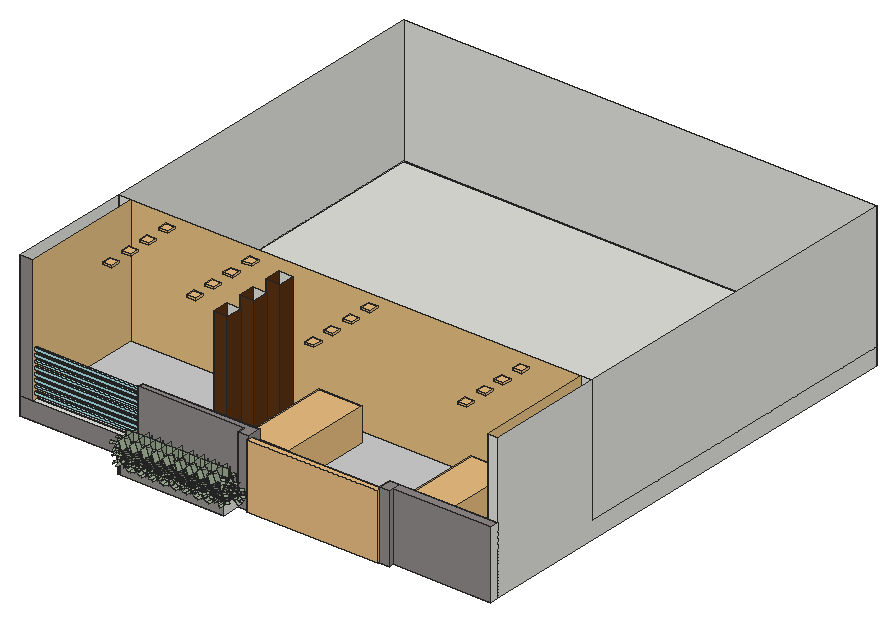
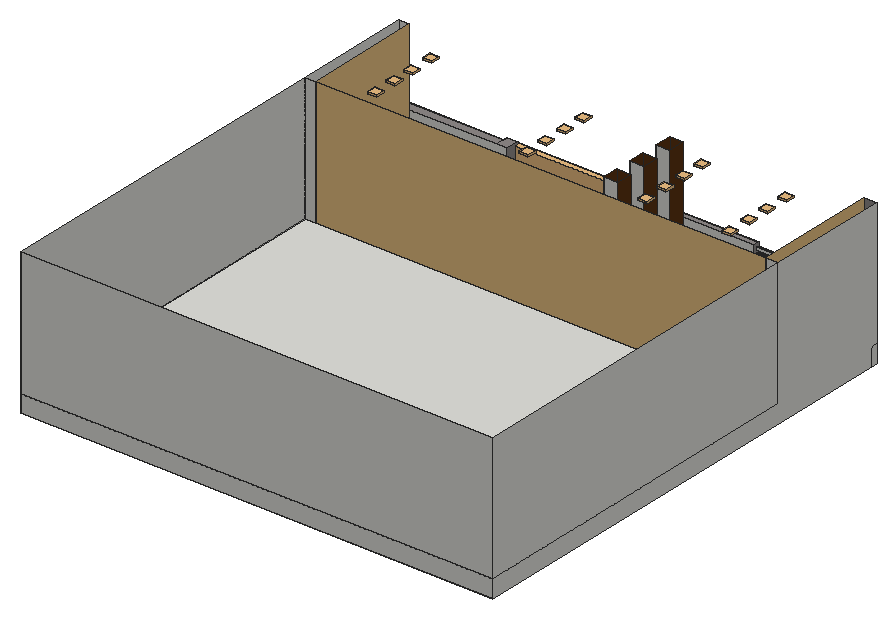
# SketchUp Ruby script. Lengths in inches.
U = 1.inch
M = Sketchup.active_model
def pt(a) = Geom::Point3d.new(a.map { |v| v * U })
def face(e, loops, mat)
  f = e.add_face(loops[0].map { |a| pt(a) })
  loops[1..].each { |l| e.add_face(l.map { |a| pt(a) }).erase! }
  f.material = f.back_material = mat if mat
  f
end
# faces: each face lists its corners as indices into pts; further lists are holes
def faces(e, pts, list, mat = nil) = list.each { |f| face(e, (f[0].is_a?(Array) ? f : [f]).map { |l| l.map { |i| pts[i] } }, mat) }
# xy, xz, yz: faces in a plane at the given z, y or x. An outline is a flat list of corners, or four numbers for a rectangle; further outlines are holes
def ring(l) = l.size == 4 ? [[l[0], l[1]], [l[2], l[1]], [l[2], l[3]], [l[0], l[3]]] : l.each_slice(2).to_a
def flat(e, list, mat, &to3) = list.each { |f| face(e, (f[0].is_a?(Array) ? f : [f]).map { |l| ring(l).map { |u, v| to3.(u, v) } }, mat) }
def xy(e, z, list, mat = nil) = flat(e, list, mat) { |x, y| [x, y, z] }
def xz(e, y, list, mat = nil) = flat(e, list, mat) { |x, z| [x, y, z] }
def yz(e, x, list, mat = nil) = flat(e, list, mat) { |y, z| [x, y, z] }
def lines(e, pts, list) = list.each { |a, b| e.add_line(pt(pts[a]), pt(pts[b])) }
# prism: a flat outline (further loops are holes) pulled along v
def prism(e, loops, v, mat = nil)
  f = face(e, loops, mat); d = Geom::Vector3d.new(v.map { |x| x * U })
  f.pushpull(f.normal.samedirection?(d) ? d.length : -d.length)
end
def box(e, o, s, mat = nil) = prism(e, [[o, [o[0] + s[0], o[1], o[2]], [o[0] + s[0], o[1] + s[1], o[2]], [o[0], o[1] + s[1], o[2]]]], [0, 0, s[2]], mat)
def at(x, y, z, deg = 0) = Geom::Transformation.translation(pt([x, y, z])) * Geom::Transformation.rotation(ORIGIN, Z_AXIS, deg.degrees)
def axes(o, x, y, z) = Geom::Transformation.new([*x, 0, *y, 0, *z, 0, *pt(o).to_a, 1])
def part(name) = M.definitions.add(name)
# library, detail: a bought-in or finely detailed component or shape, given as its bounding box
def library(name, o, s) = part(name).tap { |d| box(d.entities, o, s) }
def detail(e, o, s) = box(e.add_group.entities, o, s)
def put(e, d, t, mat = nil) = e.add_instance(d, t).tap { |i| i.material = mat if mat }
def group(e, t, mat = nil) = e.add_group.tap { |g| g.transformation = t; g.material = mat if mat }.entities
root = M.entities
M.materials.add("Generic").color = [90, 50, 18]
M.materials.add("Generic\#5").color = [233, 194, 132]
M.materials.add("Generic\#7").color = [171, 227, 232]
M.materials.add("[Carrera Marble]").color = [207, 207, 207]
M.materials.add("[Granite Light Gray]").color = [149, 148, 144]
M.materials.add("[Stone Marble]").color = [143, 138, 136]
M.materials.add("hymenocallis littoralis").color = [156, 172, 146]
c1 = part("Group\#856")
xy(c1.entities,7.38,[[0,0,5.5,15.91]],"hymenocallis littoralis")
p = [[5.5,28.78,0],[5.5,26.79,3.44],[0,26.79,3.44],[0,28.78,0],[0,23.75,6],[5.5,23.75,6],
  [0,15.91,7.38],[5.5,15.91,7.38]]
faces(c1.entities,p,[[0,1,2,3],[4,2,1,5],[6,4,5,7]],"hymenocallis littoralis")
c2 = part("Group\#854")
xy(c2.entities,7.38,[[0,0,5.5,15.91],[0,15.91,5.5,23.87]],"hymenocallis littoralis")
p = [[5.5,31.07,4.3],[5.5,27.74,6.47],[0,27.74,6.47],[0,31.07,4.3],[0,23.87,7.38],[5.5,23.87,7.38]]
faces(c2.entities,p,[[0,1,2,3],[4,2,1,5]],"hymenocallis littoralis")
c3 = part("Group\#857")
xy(c3.entities,7.38,[[0,0,5.6,15.91]],"hymenocallis littoralis")
p = [[5.6,28.78,0],[5.6,26.79,3.44],[0,26.79,3.44],[0,28.78,0],[0,23.75,6],[5.6,23.75,6],
  [0,15.91,7.38],[5.6,15.91,7.38]]
faces(c3.entities,p,[[0,1,2,3],[4,2,1,5],[6,4,5,7]],"hymenocallis littoralis")
c4 = part("Group\#855")
put(c4.entities,c2,axes([6.09,8.57,-0.52],[0.446,0.85617,0.26089],[-0.18444,-0.19731,0.96283],[0.87582,-0.47754,0.0699]))
put(c4.entities,c2,axes([6.29,7.28,-1.71],[0.37058,0.92707,-0.05667],[-0.32382,0.19004,0.99128],[0.87712,-0.32925,0.34964]))
put(c4.entities,c2,axes([11.04,16.14,-0.7],[1,0,0],[0,0.16628,1.02662],[0,-1.18456,0.19186]))
c5 = part("Group\#860")
put(c5.entities,c1,axes([24.57,32.05,-1.76],[0.9552,-0.22102,-0.19681],[0.4036,0.95545,0.88585],[-0.00568,-0.67859,0.7345]))
put(c5.entities,c1,axes([23.95,29.24,-2.4],[0,1,0],[-0.76041,0,0.64945],[0.64945,0,0.76041]))
put(c5.entities,c1,axes([24.22,24.72,-0.48],[-0.70711,0.70711,0],[-0.32757,-0.32757,0.80237],[0.61237,0.61237,0.5]))
put(c5.entities,c2,axes([20.66,37.22,-0.63],[1.12361,0.03262,0.39091],[-0.43499,0.29739,0.78777],[0.09852,-1.27434,0.37535]))
put(c5.entities,c1,axes([28.75,24.45,-2.4],[-1,0,0],[0,-0.76041,0.64945],[0,0.64945,0.76041]))
put(c5.entities,c3,axes([30.4,30.98,-3.7],[0.65676,-0.72002,0.22414],[0.55667,0.66341,0.5],[-0.50871,-0.20361,0.83652]))
put(c5.entities,c3,axes([32.41,29.61,-3.7],[0.04029,-0.97372,0.22414],[0.85287,0.15038,0.5],[-0.52057,0.17102,0.83652]))
put(c5.entities,c1,axes([31.89,25.85,-1.76],[-0.92056,0.33739,-0.19681],[-0.5186,-0.89824,0.88585],[0.08952,0.67268,0.7345]))
put(c5.entities,c1,axes([25.55,34.78,-0.48],[0.86603,0.5,0],[-0.25,0.43301,0.86603],[0.43301,-0.75,0.5]))
put(c5.entities,c3,axes([20.4,16.9375,-8.07],[-0.70711,0.70711,0],[-0.35754,-0.35754,0.65422],[1.3987,1.3987,1.52882]))
put(c5.entities,c1,axes([32.86,34.14,-0.48],[0.76604,-0.64279,0],[0.32139,0.38302,0.86603],[-0.55667,-0.66341,0.5]))
put(c5.entities,c1,axes([27.15,34.7,-0.1],[0.82472,-0.17528,-0.53769],[0.53769,0.53769,0.64945],[0.17528,-0.82472,0.53769]))
put(c5.entities,c1,axes([33.58,28.77,-2.4],[0,-1,0],[0.76041,0,0.64945],[-0.64945,0,0.76041]))
put(c5.entities,c1,axes([26.43,23.87,-2.81],[-0.75126,0.04415,0.65853],[0.53769,-0.53769,0.64945],[0.38276,0.84199,0.3802]))
put(c5.entities,c1,axes([28.78,23.98,-2.4],[-1,0,0],[0,-0.76041,0.64945],[0,0.64945,0.76041]))
put(c5.entities,c1,axes([25.39,25.38,-2.4],[-0.70711,0.70711,0],[-0.53769,-0.53769,0.64945],[0.45923,0.45923,0.76041]))
put(c5.entities,c1,axes([27.32,21.63,-0.1],[-0.45923,0.70711,-0.53769],[-0.76041,0,0.64945],[0.45923,0.70711,0.53769]))
put(c5.entities,c1,axes([25.17,27.625,-1.76],[0.56416,0.80187,-0.19681],[-0.66673,0.66673,0.80532],[0.62659,-0.26057,0.7345]))
put(c5.entities,c3,axes([27.59,27.04,-3.96],[-0.8993,-0.06127,0.43301],[0.2962,-0.8138,0.5],[0.32175,0.57791,0.75]))
put(c5.entities,c3,axes([26.98,24.5,-3.18],[-0.5,0.86603,0],[-0.75,-0.43301,0.5],[0.43301,0.25,0.86603]))
put(c5.entities,c3,axes([24.55,27.74,-3.7],[0.29517,0.92878,0.22414],[-0.85287,0.15038,0.5],[0.43068,-0.33875,0.83652]))
put(c5.entities,c3,axes([24.26,29.8,-3.18],[0.76604,0.64279,0],[-0.47317,0.5639,0.425],[0.32139,-0.38302,0.86603]))
put(c5.entities,c3,axes([25.98,32.46,-3.18],[1,0,0],[0,0.86603,0.5],[0,-0.5,0.86603]))
put(c5.entities,c1,axes([28.78,33.57,-2.4],[1,0,0],[0,0.76041,0.64945],[0,-0.64945,0.76041]))
put(c5.entities,c4,at(14.99,21.38,2.5))
put(c5.entities,c2,axes([34.63,26.34,-1.46],[-0.70089,-0.70877,0.07994],[0.4756,-0.38088,0.79293],[-0.53156,0.59378,0.60405]))
put(c5.entities,c2,axes([28.14,16.92,1.8125],[-1.19719,0.6912,0],[-0.09607,-0.16641,0.94244],[0.68444,1.18549,0.17613]))
put(c5.entities,c2,axes([31.5625,35.84,0.97],[0.66765,-1.1564,0.35779],[0.04445,0.30732,0.91033],[-1.20828,-0.64496,0.17012]))
put(c5.entities,c2,axes([38.94,22.51,0.89],[-0.97932,-0.67164,-0.05202],[0.27787,-0.41401,0.90999],[-0.85985,0.93577,0.32097]))
put(c5.entities,c2,axes([38.44,21.09,1.98],[-1.02864,-0.54856,0.2395],[0.33481,0.06999,0.88388],[-0.77261,1.08328,0.06417]))
put(c5.entities,c3,axes([35.02,30.51,-1.3],[-0.17365,-0.98481,0],[0.60224,-0.10619,0.79122],[-0.7792,0.13739,0.61153]))
put(c5.entities,c3,axes([29.41,22.33,-1.3],[-0.93969,0.34202,0],[-0.20915,-0.57465,0.79122],[0.27061,0.74351,0.61153]))
put(c5.entities,c2,axes([19.64,36,-1.62],[1.18194,0.09546,0.08234],[-0.14377,0.68823,0.76313],[0.21457,-1.1326,0.62386]))
put(c5.entities,c3,axes([24.25,24.14,-1.3],[-0.34202,0.93969,0],[-0.57465,-0.20915,0.79122],[0.74351,0.27061,0.61153]))
put(c5.entities,c3,axes([25.98,34.61,-1.3],[1,0,0],[0,0.61153,0.79122],[0,-0.79122,0.61153]))
put(c5.entities,c3,axes([31.16,34.41,-1.64],[0.56518,-0.80224,-0.19234],[0.73413,0.34233,0.72935],[-0.47639,-0.50772,0.71782]))
put(c5.entities,c3,axes([40.52,26.84,-5.82],[-0.42262,-0.90631,0],[0.48019,-0.22391,0.68552],[-1.43418,0.66877,1.22305]))
put(c5.entities,c1,axes([29.86,38.42,-1.01],[0.89064,-0.37013,0.26413],[-0.03924,0.63286,1.01918],[-0.45353,-0.76487,0.45748]))
put(c5.entities,c1,axes([29.34,22.4,-0.48],[-0.99619,-0.08716,0],[0.04358,-0.4981,0.86603],[-0.07548,0.86273,0.5]))
c6 = part("Group\#858")
xz(c6.entities,10.07,[[9.07,0,10.07,31.01],[0,31.01,0,45.12,20.13,45.12,20.13,31.01,10.07,31.01,10.07,32.58,9.07,32.58,9.07,31.01]],"hymenocallis littoralis")
yz(c6.entities,10.07,[[0,31.01,20.13,45.12]],"hymenocallis littoralis")
p = [[9.57,9.2,0],[10.07,10.07,0],[10.07,10.07,31.01],[10.07,10.07,32.58],[9.57,9.2,32.58]]
faces(c6.entities,p,[[0,1,2,3,4]],"hymenocallis littoralis")
c7 = part("cây lá nắng")
put(c7.entities,c5,axes([49.26,-2.75,0],[0.63109,0.63109,0],[-0.63109,0.63109,0],[0,0,0.935]))
g1 = group(c7.entities,at(26.6,-8.68,0))
put(g1,c1,axes([-4.72,35.73,-1.65],[0.74231,0.46334,-0.18402],[-0.34827,0.85768,0.82827],[0.42467,-0.43184,0.68675]))
put(g1,c1,axes([-3.34,33.57,-2.24],[-0.63109,0.63109,0],[-0.47989,-0.47989,0.60723],[0.40986,0.40986,0.71098]))
put(g1,c1,axes([-0.3125,30.89,-0.45],[-0.8925,0,0],[0,-0.41345,0.75022],[0,0.77293,0.4675]))
put(g1,c2,axes([-10.79,39.66,-0.59],[0.68852,0.72969,0.3655],[-0.4622,-0.08684,0.73657],[0.86641,-0.74205,0.35095]))
put(g1,c1,axes([2.71,33.57,-2.24],[-0.63109,-0.63109,0],[0.47989,-0.47989,0.60723],[-0.40986,0.40986,0.71098]))
put(g1,c3,axes([-0.37,38.74,-3.46],[0.86887,-0.03992,0.20957],[-0.06737,0.76999,0.4675],[-0.19255,-0.44954,0.78214]))
put(g1,c3,axes([1.76,39.14,-3.46],[0.63993,-0.58908,0.20957],[0.44333,0.63315,0.4675],[-0.43646,-0.2206,0.78214]))
put(g1,c1,axes([3.81,36.4375,-1.65],[-0.79389,-0.36803,-0.18402],[0.23959,-0.89415,0.82827],[-0.36803,0.48102,0.68675]))
put(g1,c1,axes([-5.83,38.07,-0.45],[0.231,0.86209,0],[-0.43104,0.1155,0.80973],[0.74659,-0.20005,0.4675]))
put(g1,c3,axes([2.18,23.5625,-7.55],[-0.8925,0,0],[0,-0.45128,0.6117],[0,1.76542,1.42944]))
put(g1,c1,axes([-0.8125,42.28,-0.45],[0.8891,0.07779,0],[-0.03889,0.44455,0.80973],[0.06737,-0.76999,0.4675]))
put(g1,c1,axes([-4.76,39.03,-0.09],[0.63109,0.40986,-0.50274],[0,0.67866,0.60723],[0.63109,-0.40986,0.50274]))
put(g1,c1,axes([3.03,39.35,-2.24],[0.63109,-0.63109,0],[0.47989,0.47989,0.60723],[-0.40986,-0.40986,0.71098]))
put(g1,c1,axes([1.61,31.74,-2.625],[-0.50198,-0.44625,0.61573],[0.67866,0,0.60723],[-0.28982,0.77293,0.35549]))
put(g1,c1,axes([3.03,33.3,-2.24],[-0.63109,-0.63109,0],[0.47989,-0.47989,0.60723],[-0.40986,0.40986,0.71098]))
put(g1,c1,axes([0.01,32.04,-2.24],[-0.8925,0,0],[0,-0.67866,0.60723],[0,0.57963,0.71098]))
put(g1,c1,axes([3.59,30.89,-0.09],[-0.73607,0.15643,-0.50274],[-0.47989,-0.47989,0.60723],[-0.15643,0.73607,0.50274]))
put(g1,c1,axes([-1.55,33.32,-1.65],[-0.15002,0.86209,-0.18402],[-0.84154,0,0.75297],[0.55988,0.231,0.68675]))
put(g1,c3,axes([0.35,34.48,-3.71],[-0.52887,-0.60621,0.40487],[0.70051,-0.32665,0.4675],[-0.16166,0.56777,0.70125]))
put(g1,c3,axes([2.61,39.13,-1.74],[-0.86209,0.231,0],[-0.23031,-0.85954,0.15531],[0.03162,0.11799,0.91645]))
put(g1,c3,axes([-2.02,33,-3.46],[-0.39986,0.77243,0.20957],[-0.63315,-0.44333,0.4675],[0.48558,0.05802,0.78214]))
put(g1,c3,axes([-3.49,34.12,-2.97],[0.07779,0.8891,0],[-0.65449,0.05726,0.39737],[0.44455,-0.03889,0.80973]))
put(g1,c3,axes([-4.09,36.88,-2.97],[0.63109,0.63109,0],[-0.54654,0.54654,0.4675],[0.31555,-0.31555,0.80973]))
put(g1,c1,axes([-3.02,39.35,-2.24],[0.63109,0.63109,0],[-0.47989,0.47989,0.60723],[0.40986,-0.40986,0.71098]))
put(g1,c4,axes([-4.03,22.95,2.33],[0.63109,0.63109,0],[-0.63109,0.63109,0],[0,0,0.935]))
put(g1,c2,axes([5.24,38.48,-1.37],[0.00497,-0.88963,0.07474],[0.54052,0.05978,0.74139],[-0.71019,0.03927,0.56479]))
put(g1,c2,axes([7.08,28.4375,1.7],[-1.19175,-0.31933,0],[0.04439,-0.16565,0.88118],[-0.31621,1.1801,0.16468]))
put(g1,c2,axes([-2.7,42.54,0.91],[1.15114,-0.30845,0.33454],[-0.1659,0.22199,0.85115],[-0.3555,-1.16957,0.15907]))
put(g1,c2,axes([10.37,38.78,0.83],[-0.19417,-1.04191,-0.04864],[0.43664,-0.08592,0.85084],[-1.1332,0.04791,0.30011]))
put(g1,c2,axes([10.95,37.5625,1.85],[-0.30298,-0.99536,0.22393],[0.16713,0.25547,0.82643],[-1.17124,0.19607,0.06]))
put(g1,c3,axes([2.84,41.36,-1.22],[0.51192,-0.73109,0],[0.44708,0.31305,0.73979],[-0.57846,-0.40504,0.57178]))
put(g1,c3,axes([4.47,32.65,-1.22],[-0.80888,-0.37719,0],[0.23066,-0.49465,0.73979],[-0.29844,0.64,0.57178]))
put(g1,c2,axes([-10.32,35.12,-1.51],[0.68567,0.80616,0.07699],[-0.52507,0.3436,0.71352],[0.85019,-0.57936,0.58331]))
put(g1,c3,axes([0.07,30.54,-1.22],[-0.80888,0.37719,0],[-0.23066,-0.49465,0.73979],[0.29844,0.64,0.57178]))
put(g1,c3,axes([-5.45,38.24,-1.22],[0.63109,0.63109,0],[-0.38593,0.38593,0.73979],[0.49934,-0.49934,0.57178]))
put(g1,c3,axes([-2.05,41.38,-1.53],[0.86296,-0.14961,-0.17984],[0.24726,0.67935,0.68194],[0.01977,-0.62107,0.67116]))
put(g1,c3,axes([8.63,42.51,-5.4375],[0.30525,-0.83868,0],[0.44435,0.16173,0.64096],[-1.32716,-0.48305,1.14356]))
put(g1,c1,axes([-5.4,43.09,-0.94],[0.79566,0.32849,0.24696],[-0.42416,0.37462,0.95293],[0.19648,-0.76892,0.42774]))
put(g1,c1,axes([4.38,32.65,-0.45],[-0.57369,-0.68369,0],[0.34185,-0.28684,0.80973],[-0.5921,0.49683,0.4675]))
put(g1,c3,axes([-2,33.84,-0.15],[-0.24601,0.85793,0],[-0.85539,-0.24528,0.15531],[0.11742,0.03367,0.91645]))
put(g1,c3,axes([0.17,30.83,-4.47],[-0.24601,0.85793,0],[-0.85539,-0.24528,0.15531],[0.11742,0.03367,0.91645]))
put(g1,c3,axes([-1.97,32.18,-4.47],[0.58524,0.67383,0],[-0.67184,0.58351,0.15531],[0.09222,-0.0801,0.91645]))
put(g1,c3,axes([-2,34.71,-4.47],[0.88392,-0.12346,0],[0.12309,0.88131,0.15531],[-0.0169,-0.12098,0.91645]))
put(g1,c3,axes([0.11,36.12,-4.47],[0.37822,-0.8084,0],[0.80601,0.37711,0.15531],[-0.11064,-0.05177,0.91645]))
put(c7.entities,c6,axes([29.71,14.29,6.94],[0.425,0.73612,0],[-0.6771,0.39092,-0.33349],[-0.26859,0.15507,0.72712]))
put(c7.entities,c6,axes([42.0625,26.12,6.94],[0.85,0,0],[0,0.78185,-0.33349],[0,0.33349,0.78185]))
put(c7.entities,c5,axes([7.3125,23.0625,0],[0.8925,0,0],[0,0.8925,0],[0,0,0.935]))
put(c7.entities,c6,axes([24.4375,40.23,2.05],[0.85,0,0],[0,0.85,0],[0,0,0.85]))
c8 = part("Planting+101")
put(c8.entities,c7,axes([21.34,32.96,-4.59],[0,-0.71,0],[-0.71,0,0],[0,0,0.71]))
c9 = library("Group\#32",[0,0,0],[139.4,5.58,74.57])
c10 = library("2016+Honda+Civic+LX+Sedan",[0.01,0.03,0.02],[16.17,34.46,10.62])
c11 = library("Tlon Light 450 Ceiling 152 006",[-8.86,-8.86,-3.78],[17.72,17.72,3.56])
xy(root,-33.9375,[[128.25,8.25,128.25,34.9375,2.3125,34.9375,2.3125,41,253.16,41,253.16,26.8125,241.72,26.8125,241.72,8.25],[392.56,26.8125,392.56,41,507.875,41,507.875,31.5625,403.43,31.5625,403.43,26.8125],[2.3125,41,507.875,546.8125]])
xy(root,-33.5625,[[129.53,9.53,240.4375,33.66]])
xy(root,-23.25,[[[128.25,8.25,241.72,34.9375],[129.53,9.53,240.4375,33.66]]])
xy(root,-15.1875,[[2.3125,34.9375,15.4375,41],[15.4375,34.9375,128.25,41],[2.3125,166.1875,507.875,546.8125]])
xy(root,-15.1875,[[[15.4375,41,497,166.1875],[190.6,127.93,205.29,145.49],[190.6,92.87,205.29,110.43],[190.6,57.81,205.29,75.37]]],"[Carrera Marble]")
xy(root,-9.21,[[14.19,36.38,128.25,39.01]])
xy(root,-6.58,[[14.19,36.38,128.25,39.01]],"Generic\#7")
xy(root,-3.21,[[14.19,36.38,128.25,39.01]])
xy(root,-0.58,[[14.19,36.38,128.25,39.01]],"Generic\#7")
xy(root,2.79,[[14.19,36.38,128.25,39.01]])
xy(root,5.42,[[14.19,36.38,128.25,39.01]],"Generic\#7")
xy(root,8.79,[[14.19,36.38,128.25,39.01]])
xy(root,11.42,[[14.19,36.38,128.25,39.01]],"Generic\#7")
xy(root,14.79,[[14.19,36.38,128.25,39.01]])
xy(root,17.42,[[14.19,36.38,128.25,39.01]],"Generic\#7")
xy(root,20.79,[[14.19,36.38,128.25,39.01]])
xy(root,23.42,[[14.19,36.38,128.25,39.01]],"Generic\#7")
xy(root,26.79,[[14.19,36.38,128.25,39.01]])
xy(root,29.42,[[14.19,36.38,128.25,39.01]],"Generic\#7")
xy(root,32.79,[[14.19,36.38,128.25,39.01]])
xy(root,35.42,[[14.19,36.38,128.25,39.01]],"Generic\#7")
xy(root,38.3125,[[241.72,26.8125,253.16,26.8125,253.16,41,128.25,41,128.25,34.9375,241.72,34.9375],[392.56,26.8125,403.43,41],[403.43,31.5625,507.875,41]],"[Stone Marble]")
xz(root,8.25,[[128.25,-33.9375,241.72,-23.25]],"[Granite Light Gray]")
xz(root,9.53,[[129.53,-33.5625,240.4375,-23.25]])
xz(root,26.8125,[[241.72,-33.9375,253.16,38.3125],[392.56,-33.9375,403.43,38.3125]],"[Stone Marble]")
xz(root,31.5625,[[403.43,-33.9375,507.875,38.3125]],"[Stone Marble]")
xz(root,33.66,[[129.53,-33.5625,240.4375,-23.25]])
xz(root,34.9375,[[2.3125,-33.9375,128.25,-15.1875],[128.25,-23.25,241.72,38.3125],[2.3125,-15.1875,15.4375,120]],"[Stone Marble]")
xz(root,36.38,[[14.19,-9.21,128.25,-6.58],[14.19,-3.21,128.25,-0.58],[14.19,2.79,128.25,5.42],[14.19,8.79,128.25,11.42],[14.19,14.79,128.25,17.42],
  [14.19,20.79,128.25,23.42],[14.19,26.79,128.25,29.42],[14.19,32.79,128.25,35.42]],"Generic\#7")
xz(root,39.01,[[14.19,-9.21,128.25,-6.58],[14.19,-3.21,128.25,-0.58],[14.19,2.79,128.25,5.42],[14.19,8.79,128.25,11.42],[14.19,14.79,128.25,17.42],
  [14.19,20.79,128.25,23.42],[14.19,26.79,128.25,29.42],[14.19,32.79,128.25,35.42]])
xz(root,41,[[2.3125,-33.9375,253.16,-15.1875],[392.56,-33.9375,507.875,-15.1875],[128.25,-15.1875,253.16,38.3125],[392.56,-15.1875,497,38.3125],[497,-15.1875,507.875,38.3125],
  [497,38.3125,507.875,120]])
xz(root,41,[[253.16,-33.9375,392.56,-15.1875]],"[Carrera Marble]")
xz(root,57.81,[[190.6,-15.1875,205.29,122]],"Generic")
xz(root,75.37,[[190.6,-15.1875,205.29,122]])
xz(root,92.87,[[190.6,-15.1875,205.29,122]],"Generic")
xz(root,110.43,[[190.6,-15.1875,205.29,122]])
xz(root,127.93,[[190.6,-15.1875,205.29,122]],"Generic")
xz(root,145.49,[[190.6,-15.1875,205.29,122]])
xz(root,166.1875,[[2.3125,-15.1875,15.4375,120],[497,-15.1875,507.875,120]])
xz(root,166.1875,[[15.4375,-15.1875,497,120]],"Generic\#5")
xz(root,546.8125,[[2.3125,-33.9375,507.875,-15.1875],[2.3125,-15.1875,507.875,120]])
yz(root,2.3125,[[34.9375,-33.9375,41,-15.1875],[41,-33.9375,41,-15.1875,34.9375,-15.1875,34.9375,120,166.1875,120,166.1875,-15.1875,546.8125,-15.1875,546.8125,-33.9375],[166.1875,-15.1875,546.8125,120]])
yz(root,14.19,[[36.38,-9.21,39.01,-6.58],[36.38,-3.21,39.01,-0.58],[36.38,2.79,39.01,5.42],[36.38,8.79,39.01,11.42],[36.38,14.79,39.01,17.42],
  [36.38,20.79,39.01,23.42],[36.38,26.79,39.01,29.42],[36.38,32.79,39.01,35.42]])
yz(root,15.4375,[[34.9375,-15.1875,166.1875,120]],"Generic\#5")
yz(root,128.25,[[8.25,-33.9375,34.9375,-23.25]],"[Granite Light Gray]")
yz(root,128.25,[[[34.9375,-15.1875,41,38.3125],[36.38,-9.21,39.01,-6.58],[36.38,-3.21,39.01,-0.58],[36.38,2.79,39.01,5.42],[36.38,8.79,39.01,11.42],[36.38,14.79,39.01,17.42],[36.38,20.79,39.01,23.42],[36.38,26.79,39.01,29.42],[36.38,32.79,39.01,35.42]]],"[Stone Marble]")
yz(root,129.53,[[9.53,-33.5625,33.66,-23.25]])
yz(root,190.6,[[57.81,-15.1875,75.37,122],[92.87,-15.1875,110.43,122],[127.93,-15.1875,145.49,122]],"Generic")
yz(root,205.29,[[57.81,-15.1875,75.37,122],[92.87,-15.1875,110.43,122],[127.93,-15.1875,145.49,122]],"Generic")
yz(root,240.4375,[[9.53,-33.5625,26.8125,-23.25],[26.8125,-33.5625,33.66,-23.25]])
yz(root,241.72,[[8.25,-33.9375,26.8125,-23.25]])
yz(root,241.72,[[26.8125,-23.25,34.9375,38.3125]],"[Stone Marble]")
yz(root,253.16,[[26.8125,-33.9375,41,38.3125]],"[Stone Marble]")
yz(root,392.56,[[26.8125,-33.9375,41,38.3125]],"[Stone Marble]")
yz(root,403.43,[[26.8125,-33.9375,31.5625,38.3125]],"[Stone Marble]")
yz(root,497,[[41,-15.1875,166.1875,120]],"Generic\#5")
yz(root,507.875,[[31.5625,-33.9375,41,38.3125],[41,-33.9375,546.8125,-33.9375,546.8125,-15.1875,166.1875,-15.1875,166.1875,120,41,120],[166.1875,-15.1875,546.8125,120]])
put(root,c8,at(141.55,18.4375,-26.14))
put(root,c8,at(153.42,18.4375,-26.14))
put(root,c8,at(165.3,18.4375,-26.14))
put(root,c8,at(177.17,18.4375,-26.14))
put(root,c8,at(189.05,18.4375,-26.14))
put(root,c8,at(200.92,18.4375,-26.14))
put(root,c8,at(212.8,18.4375,-26.14))
put(root,c8,at(224.67,18.4375,-26.14))
put(root,c8,at(236.55,18.4375,-26.14))
put(root,c9,axes([253.16,24.42,-33.43],[1,0,0],[0,1,0],[0,0,0.93]))
put(root,c10,axes([228.45,53.16,-15.26],[2.8355,0,0],[0,2.8355,0],[0,0,3.28918]))
put(root,c10,axes([391.55,58.69,-15.25],[2.675,0,0],[0,2.675,0],[0,0,2.675]))
put(root,c11,axes([448.11,73.1875,119.85],[0.54664,0,0],[0,0.54664,0],[0,0,0.54664]))
put(root,c11,axes([448.11,98.5625,119.85],[0.54664,0,0],[0,0.54664,0],[0,0,0.54664]))
put(root,c11,axes([448.11,121.6875,119.85],[0.54664,0,0],[0,0.54664,0],[0,0,0.54664]))
put(root,c11,axes([448.11,146.75,119.85],[0.54664,0,0],[0,0.54664,0],[0,0,0.54664]))
put(root,c11,axes([285.09,147.73,120.25],[0.54664,0,0],[0,0.54664,0],[0,0,0.54664]))
put(root,c11,axes([285.09,123.16,120.25],[0.54664,0,0],[0,0.54664,0],[0,0,0.54664]))
put(root,c11,axes([285.09,97.91,120.25],[0.54664,0,0],[0,0.54664,0],[0,0,0.54664]))
put(root,c11,axes([285.09,73.1,120.25],[0.54664,0,0],[0,0.54664,0],[0,0,0.54664]))
put(root,c11,axes([158.09,73.1,120.25],[0.54664,0,0],[0,0.54664,0],[0,0,0.54664]))
put(root,c11,axes([158.09,97.73,120.25],[0.54664,0,0],[0,0.54664,0],[0,0,0.54664]))
put(root,c11,axes([158.09,122.35,120.25],[0.54664,0,0],[0,0.54664,0],[0,0,0.54664]))
put(root,c11,axes([158.09,147.73,120.25],[0.54664,0,0],[0,0.54664,0],[0,0,0.54664]))
put(root,c11,axes([68.65,73.1,120.25],[0.54664,0,0],[0,0.54664,0],[0,0,0.54664]))
put(root,c11,axes([68.65,98.16,120.25],[0.54664,0,0],[0,0.54664,0],[0,0,0.54664]))
put(root,c11,axes([68.65,122.1,120.25],[0.54664,0,0],[0,0.54664,0],[0,0,0.54664]))
put(root,c11,axes([68.65,147.73,120.25],[0.54664,0,0],[0,0.54664,0],[0,0,0.54664]))
